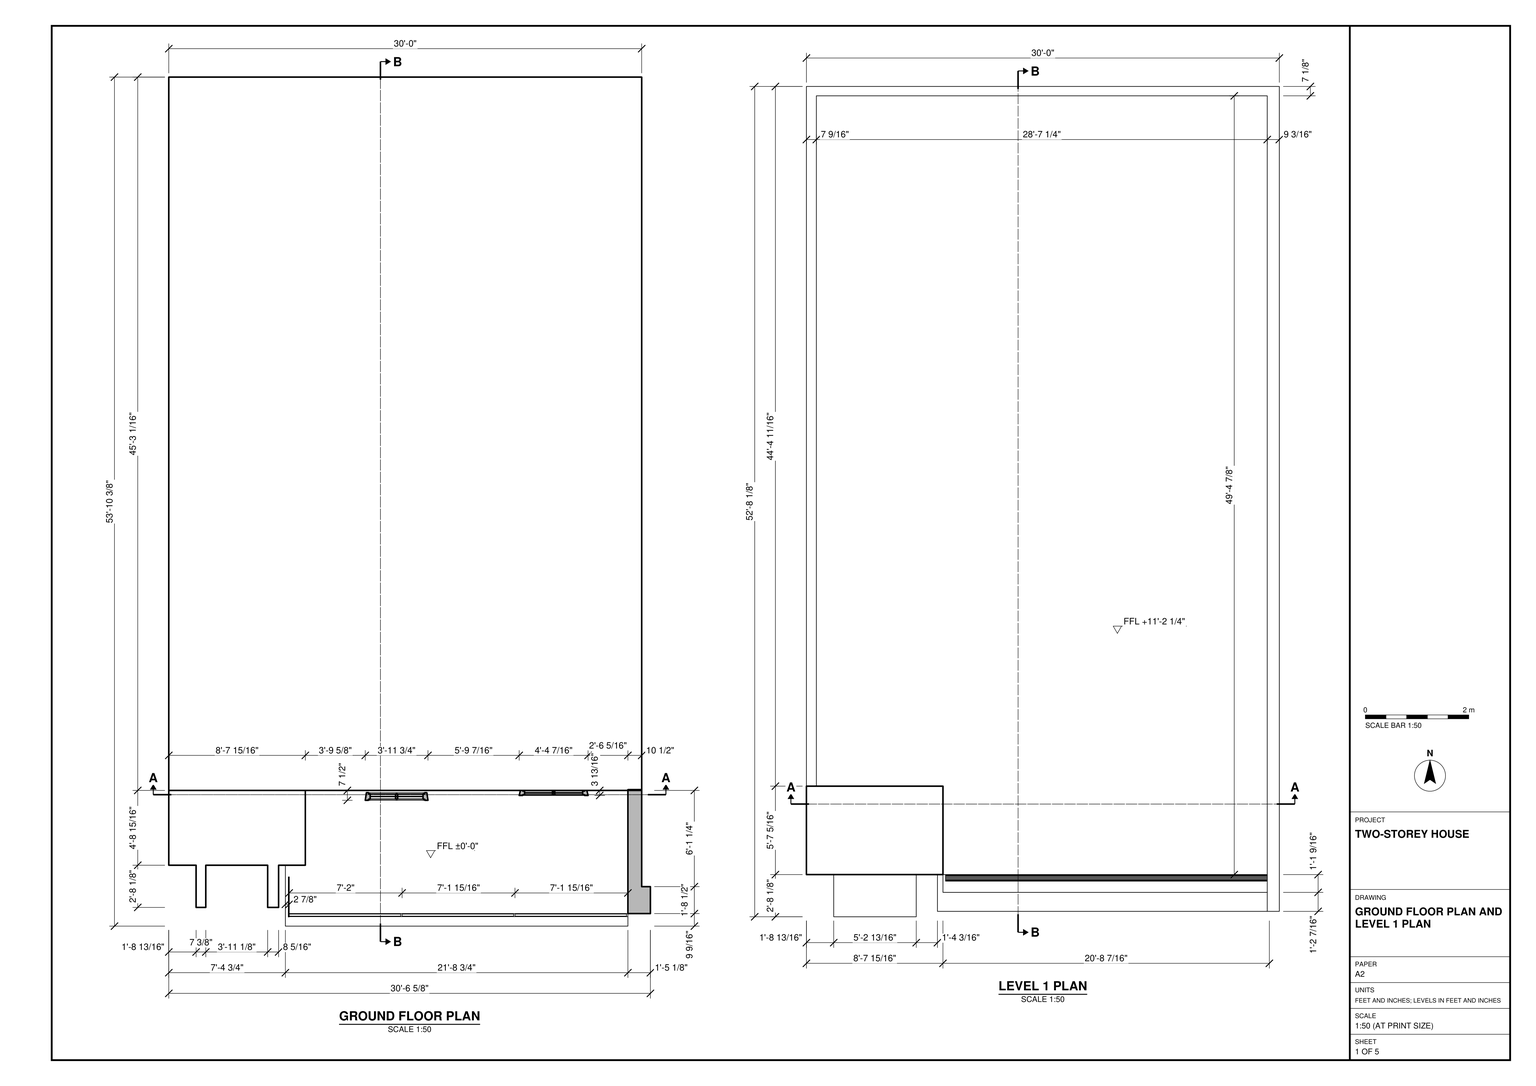
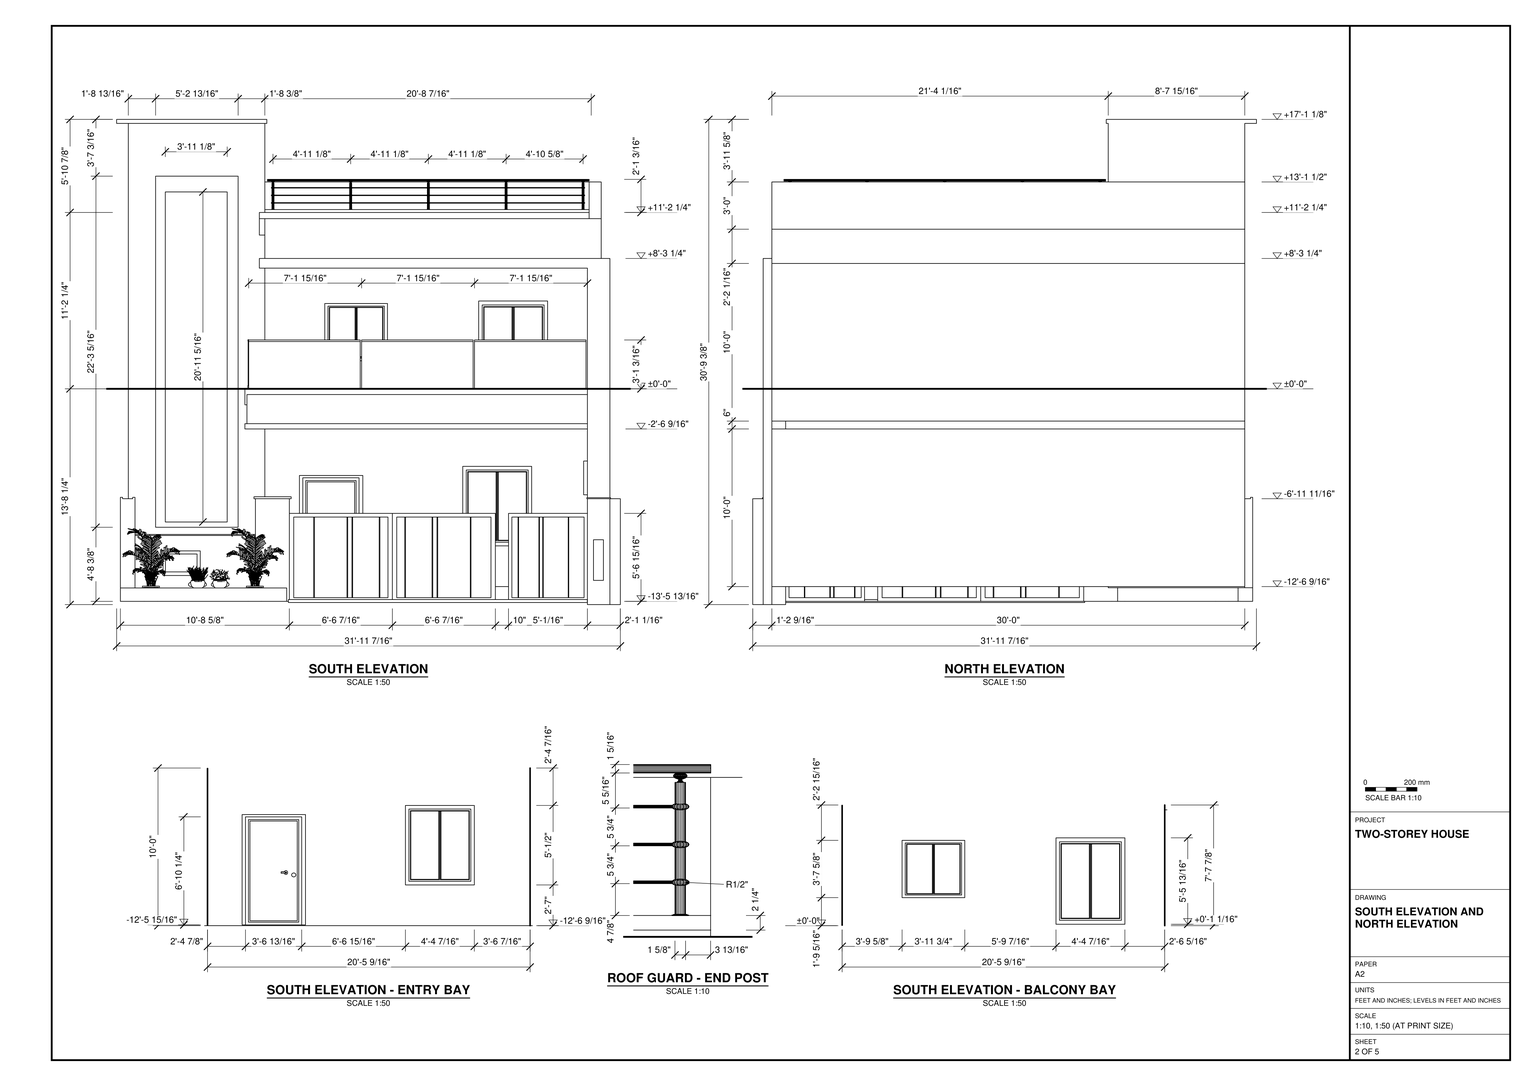
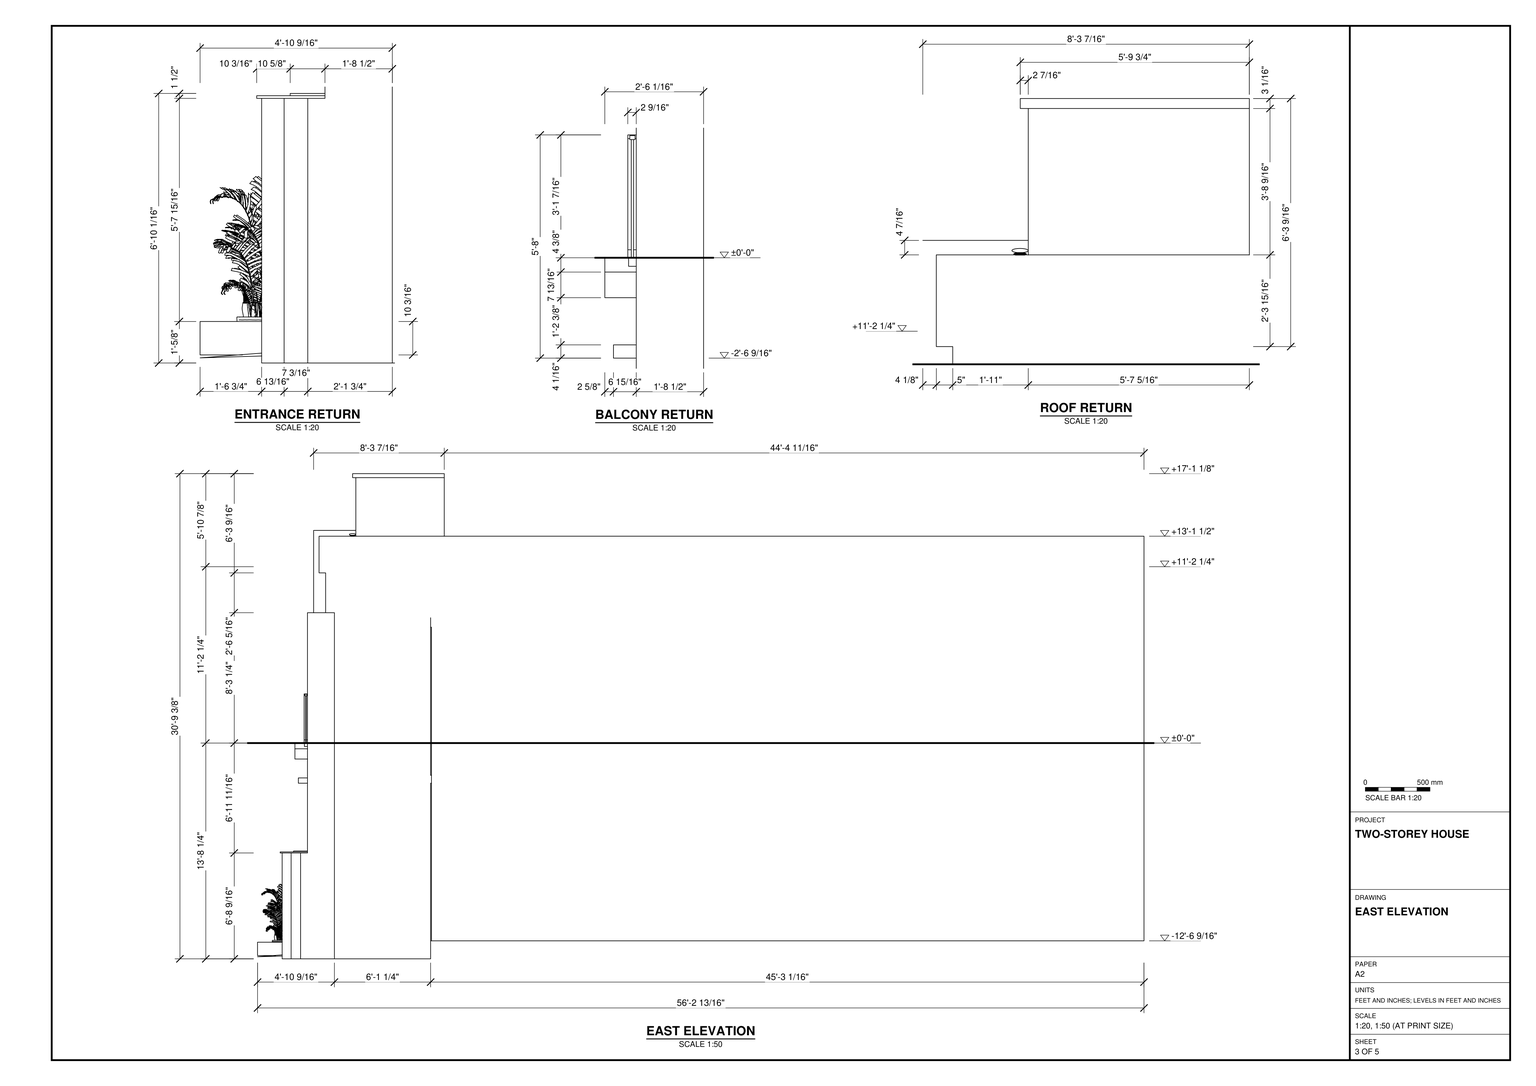
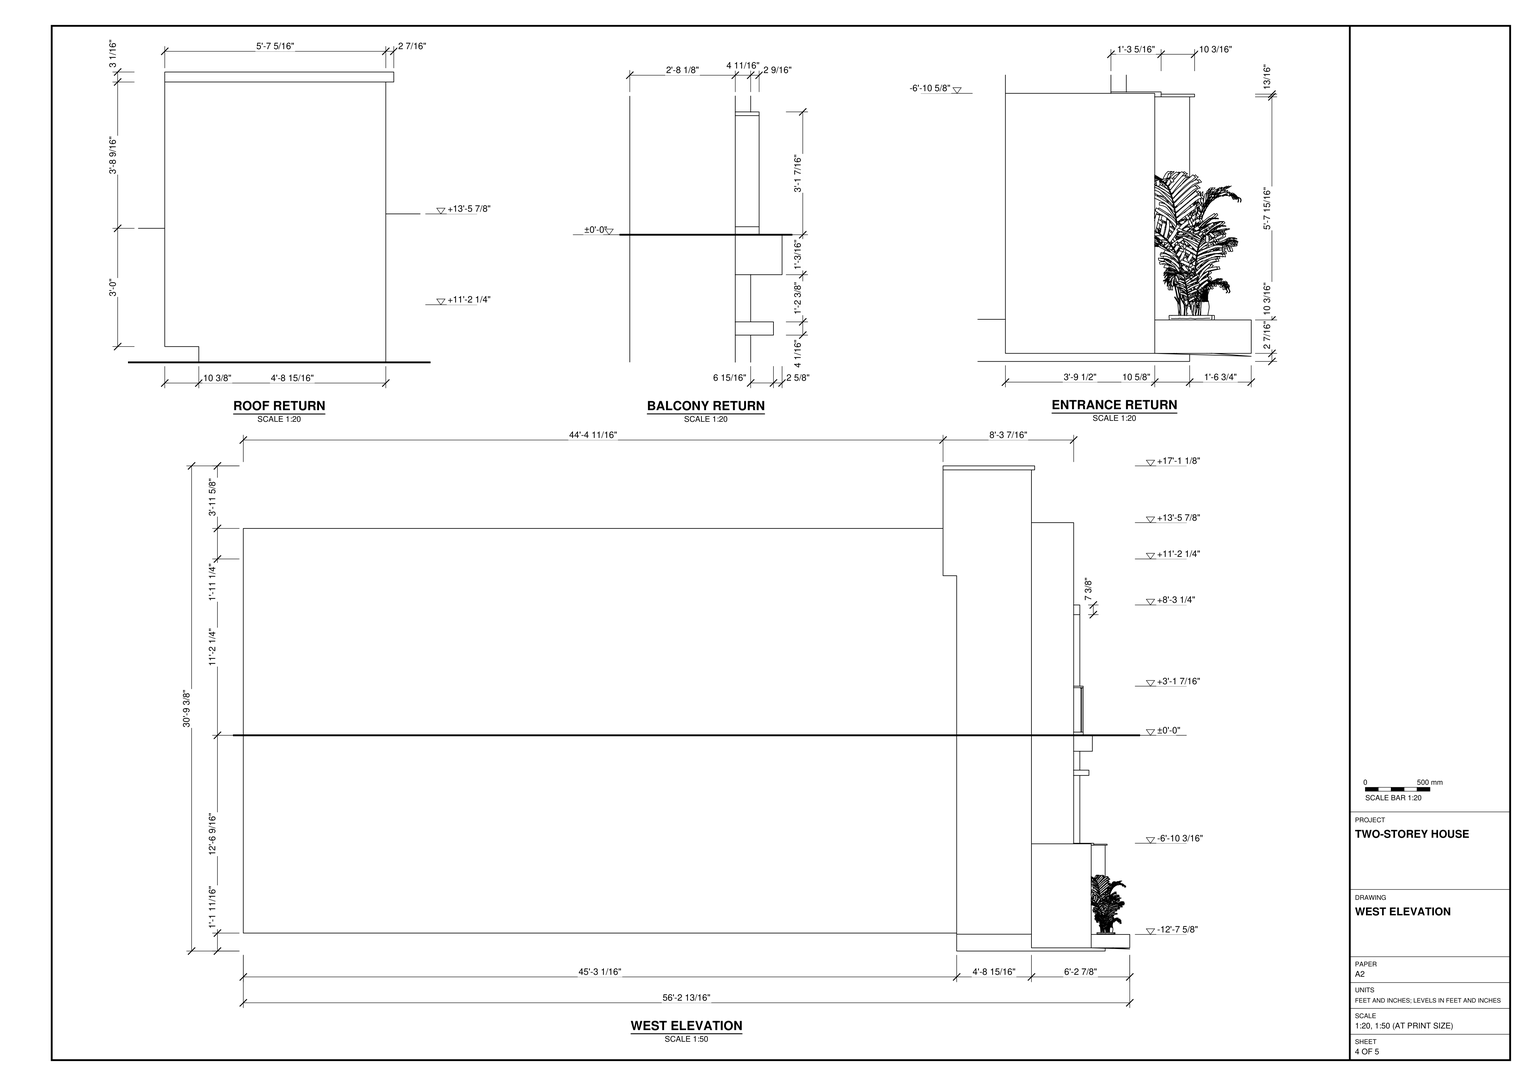
Build the two-storey house in SketchUp from task_files/diagram_01.pdf. Work in feet and inches. Set the overall width to 31'-11 7/16", the front-to-back depth to 56'-2 7/8", and the full height to 30'-9 3/8", including the projections at the entrance and roof. Use the storey levels ±0'-0" and +11'-2 1/4". Follow the elevation datums to place the lower entrance below the balcony.

Use the plans to lay out the long rectangular body, walls at their drawn thicknesses, floor slabs and flat roof with its parapet returns. On the south elevation, model the tall framed bay on the left with its inset panel and projecting cap. Beside it, place the entry door and window behind the panelled gates. Model the balcony slab, glazed guard, framed openings behind the balcony and horizontal roof guard above it. Use the return details to set the depths of these elements. Include the raised planter at the foot of the tall bay.

Keep walls, slabs, roof elements and each furniture or joinery piece shown in separate groups or components, and use components for repeated parts. Decor and loose items such as the entrance plants may be any suitable library components. Save one SketchUp model as output_files/two_storey_house_with_a_glazed_balcony_and_roof_guard.skp.

# SketchUp Ruby script. Lengths in inches.
U = 1.inch
M = Sketchup.active_model
def pt(a) = Geom::Point3d.new(a.map { |v| v * U })
def face(e, loops, mat)
  f = e.add_face(loops[0].map { |a| pt(a) })
  loops[1..].each { |l| e.add_face(l.map { |a| pt(a) }).erase! }
  f.material = f.back_material = mat if mat
  f
end
# faces: each face lists its corners as indices into pts; further lists are holes
def faces(e, pts, list, mat = nil) = list.each { |f| face(e, (f[0].is_a?(Array) ? f : [f]).map { |l| l.map { |i| pts[i] } }, mat) }
# xy, xz, yz: faces in a plane at the given z, y or x. An outline is a flat list of corners, or four numbers for a rectangle; further outlines are holes
def ring(l) = l.size == 4 ? [[l[0], l[1]], [l[2], l[1]], [l[2], l[3]], [l[0], l[3]]] : l.each_slice(2).to_a
def flat(e, list, mat, &to3) = list.each { |f| face(e, (f[0].is_a?(Array) ? f : [f]).map { |l| ring(l).map { |u, v| to3.(u, v) } }, mat) }
def xy(e, z, list, mat = nil) = flat(e, list, mat) { |x, y| [x, y, z] }
def xz(e, y, list, mat = nil) = flat(e, list, mat) { |x, z| [x, y, z] }
def yz(e, x, list, mat = nil) = flat(e, list, mat) { |y, z| [x, y, z] }
def lines(e, pts, list) = list.each { |a, b| e.add_line(pt(pts[a]), pt(pts[b])) }
# prism: a flat outline (further loops are holes) pulled along v
def prism(e, loops, v, mat = nil)
  f = face(e, loops, mat); d = Geom::Vector3d.new(v.map { |x| x * U })
  f.pushpull(f.normal.samedirection?(d) ? d.length : -d.length)
end
def box(e, o, s, mat = nil) = prism(e, [[o, [o[0] + s[0], o[1], o[2]], [o[0] + s[0], o[1] + s[1], o[2]], [o[0], o[1] + s[1], o[2]]]], [0, 0, s[2]], mat)
def at(x, y, z, deg = 0) = Geom::Transformation.translation(pt([x, y, z])) * Geom::Transformation.rotation(ORIGIN, Z_AXIS, deg.degrees)
def axes(o, x, y, z) = Geom::Transformation.new([*x, 0, *y, 0, *z, 0, *pt(o).to_a, 1])
def part(name) = M.definitions.add(name)
# library, detail: a bought-in or finely detailed component or shape, given as its bounding box
def library(name, o, s) = part(name).tap { |d| box(d.entities, o, s) }
def detail(e, o, s) = box(e.add_group.entities, o, s)
def put(e, d, t, mat = nil) = e.add_instance(d, t).tap { |i| i.material = mat if mat }
def group(e, t, mat = nil) = e.add_group.tap { |g| g.transformation = t; g.material = mat if mat }.entities
root = M.entities
M.materials.add("4WA SFSTYD G1").color = [223, 181, 107]
M.materials.add("Aluminum_Anodized_Clear\#1").color = [178, 178, 174]
M.materials.add("Aluminum_Anodized_DarkGray\#1").color = [63, 63, 63]
M.materials.add("[0029_BlanchedAlmond]").color = [255, 235, 205]
M.materials.add("[0135_DarkGray]").color = [81, 81, 81]
M.materials.add("[0136_Charcoal]").color = [35, 35, 35]
M.materials.add("[Aluminum]").color = [179, 179, 179]
M.materials.add("[Color M08]").color = [30, 30, 30]
M.materials.add("[Color M09]").color = [0, 0, 0]
M.materials.add("[Translucent Glass Gray]").color = [128, 128, 128]
M.materials["[Translucent Glass Gray]"].alpha = 0.5
M.materials.add("[Wood Cherry Original]1").color = [152, 86, 42]
M.materials.add("[Wood Floor Parquet]").color = [145, 89, 39]
M.materials.add("[Wood Floor]").color = [155, 105, 61]
M.materials.add("[Wood Lumber ButtJoined]").color = [164, 152, 112]
M.materials.add("[Wood OSB]").color = [240, 195, 122]
M.materials.add("[Wood Veneer 02]").color = [190, 128, 91]
M.materials.add("glass_architectural\#1").color = [217, 197, 188]
M.materials["glass_architectural\#1"].alpha = 0.1
M.materials.add("we3tr gdyr1").color = [92, 92, 92]
c1 = library("trol",[-1.07,-0.37,0],[9.56,15.9,13.04])
c2 = part("Cylinder08")
prism(c2.entities,[[[-163.875,-2.5,0],[-163.95,-2.96,0],[-164.16,-3.38,0],[-164.49,-3.71,0],[-164.91,-3.93,0],[-165.375,-4,0],[-165.84,-3.93,0],[-166.26,-3.71,0],[-166.59,-3.38,0],[-166.8,-2.96,0],[-166.875,-2.5,0],[-166.8,-2.04,0],[-166.59,-1.62,0],[-166.26,-1.29,0],[-165.84,-1.07,0],[-165.375,-1,0],[-164.91,-1.07,0],[-164.49,-1.29,0],[-164.16,-1.62,0],[-163.95,-2.04,0]]],[0,0,78.0625],"4WA SFSTYD G1")
c3 = library("Line04",[-167.3,-4.43,77.97],[3.85,3.86,5.82])
c4 = library("Sphere10",[-167.86,-4.99,61.78],[4.98,4.98,4.14])
c5 = part("Box01")
box(c5.entities,[-176.87,-13.55,-8.45],[462.03,13.55,8.53],"we3tr gdyr1")
c6 = part("Cylinder01")
prism(c6.entities,[[[282.23,-1.73,88.375],[282.23,-2.5,88.5],[282.23,-3.27,88.375],[282.23,-3.97,88.02],[282.23,-4.52,87.47],[282.23,-4.88,86.77],[282.23,-5,86],[282.23,-4.88,85.22],[282.23,-4.52,84.53],[282.23,-3.97,83.97],[282.23,-3.27,83.62],[282.23,-2.5,83.5],[282.23,-1.73,83.62],[282.23,-1.03,83.97],[282.23,-0.48,84.53],[282.23,-0.125,85.22],[282.23,0,86],[282.23,-0.125,86.77],[282.23,-0.48,87.47],[282.23,-1.03,88.02]]],[-455.38,0,0],"4WA SFSTYD G1")
c7 = part("Cylinder03")
prism(c7.entities,[[[-165.34,-2.03,64.49],[-165.34,-1.85,64.3125],[-165.34,-1.74,64.09],[-165.34,-1.7,63.84],[-165.34,-1.74,63.59],[-165.34,-1.85,63.37],[-165.34,-2.03,63.19],[-165.34,-2.25,63.08],[-165.34,-2.5,63.04],[-165.34,-2.75,63.08],[-165.34,-2.97,63.19],[-165.34,-3.15,63.37],[-165.34,-3.26,63.59],[-165.34,-3.3,63.84],[-165.34,-3.26,64.09],[-165.34,-3.15,64.3125],[-165.34,-2.97,64.49],[-165.34,-2.75,64.6],[-165.34,-2.5,64.64],[-165.34,-2.25,64.6]]],[438.09,0,0],"4WA SFSTYD G1")
c8 = library("Line08",[-167.875,-5,0],[5,5,0.9])
c9 = part("skp246")
put(c9.entities,c2,at(0,0,0))
put(c9.entities,c3,at(0,0,0))
put(c9.entities,c4,at(0,0,0))
put(c9.entities,c5,at(0,0,0))
put(c9.entities,c6,at(0,0,0))
put(c9.entities,c7,at(0,0,0))
put(c9.entities,c8,at(0,0,0))
put(c9.entities,c4,at(0,0,-22.16))
put(c9.entities,c4,at(0,0,-44.3))
put(c9.entities,c7,at(0,0,-22.14))
put(c9.entities,c7,at(0,0,-44.28))
put(c9.entities,c4,at(110,0,-44.3))
put(c9.entities,c4,at(110,0,-22.16))
put(c9.entities,c4,at(110,0,0))
put(c9.entities,c2,at(110,0,0))
put(c9.entities,c8,at(110,0,0))
put(c9.entities,c3,at(110,0,0))
put(c9.entities,c4,at(220,0,-22.16))
put(c9.entities,c3,at(220,0,0))
put(c9.entities,c4,at(220,0,0))
put(c9.entities,c4,at(220,0,-44.3))
put(c9.entities,c2,at(220,0,0))
put(c9.entities,c8,at(220,0,0))
put(c9.entities,c3,at(330,0,0))
put(c9.entities,c4,at(330,0,-44.3))
put(c9.entities,c4,at(330,0,-22.16))
put(c9.entities,c8,at(330,0,0))
put(c9.entities,c2,at(330,0,0))
put(c9.entities,c4,at(330,0,0))
put(c9.entities,c4,at(438.97,0,-22.16))
put(c9.entities,c4,at(438.97,0,0))
put(c9.entities,c4,at(438.97,0,-44.3))
put(c9.entities,c8,at(438.97,0,0))
put(c9.entities,c2,at(438.97,0,0))
put(c9.entities,c3,at(438.97,0,0))
c10 = part("Railing1 (1)")
put(c10.entities,c9,at(176.87,13.55,8.45))
c11 = part("window")
xy(c11.entities,-137.04,[[3.3,-12.46,3.83,49.56]],"[Wood Veneer 02]")
xy(c11.entities,-136.95,[[0,-12.36,0.53,49.45]],"[Wood Veneer 02]")
xy(c11.entities,-135.68,[[3.08,-10.98,3.3,18.15],[3.08,18.94,3.3,48.07]],"[Color M09]")
xy(c11.entities,-135.5,[[0.53,-10.78,0.74,18.05],[0.53,19.04,0.74,47.88]],"[Color M09]")
xy(c11.entities,-135.27,[[0.74,-10.54,1.91,17.37],[1.91,-10.54,3.08,17.37],[0.74,19.73,1.91,47.63],[1.91,19.73,3.08,47.63]],"[Color M09]")
xy(c11.entities,-74.87,[[1.91,17.37,3.08,19.73],[0.74,19.73,1.91,47.63]])
xy(c11.entities,-74.87,[[0.74,-10.54,1.91,17.37],[1.91,-10.54,3.08,17.37],[1.91,19.73,3.08,47.63]],"[Color M09]")
xy(c11.entities,-74.65,[[0.53,19.04,0.74,47.88]])
xy(c11.entities,-74.65,[[0.53,-10.78,0.74,18.05]],"[Color M09]")
xy(c11.entities,-74.47,[[3.08,18.15,3.3,18.94]])
xy(c11.entities,-74.47,[[3.08,-10.98,3.3,18.15],[3.08,18.94,3.3,48.07]],"[Color M09]")
xy(c11.entities,-73.2,[[0,-12.36,0.53,49.45]],"[Wood Veneer 02]")
xy(c11.entities,-73.1,[[3.3,-12.46,3.83,49.56]],"[Wood Veneer 02]")
xy(c11.entities,3.5,[[3.3,3.5,3.83,65.52]],"[Wood Veneer 02]")
xy(c11.entities,3.6,[[0,3.6,0.53,65.41]],"[Wood Veneer 02]")
xy(c11.entities,4.98,[[3.08,4.98,3.3,34.12],[3.08,34.9,3.3,64.04]],"[Color M09]")
xy(c11.entities,5.18,[[0.53,5.18,0.74,34.01],[0.53,35,0.74,63.84]],"[Color M09]")
xy(c11.entities,5.42,[[0.74,5.42,1.91,33.33],[1.91,5.42,3.08,33.33],[0.74,35.69,1.91,63.59],[1.91,35.69,3.08,63.59]],"[Color M09]")
xy(c11.entities,25.89,[[6.71,-150.99,7.52,-94.56]],"[Wood Veneer 02]")
xy(c11.entities,25.96,[[1.71,-150.9,2.52,-94.65]],"[Wood Veneer 02]")
xy(c11.entities,26.87,[[6.39,-149.64,6.71,-123.13],[6.39,-122.42,6.71,-95.9]],"[Color M09]")
xy(c11.entities,27,[[2.52,-149.46,2.84,-123.22],[2.52,-122.32,2.84,-96.08]],"[Color M09]")
xy(c11.entities,27.16,[[2.84,-149.24,4.61,-123.85],[4.61,-149.24,6.39,-123.85],[2.84,-121.7,4.61,-96.31],[4.61,-121.7,6.39,-96.31]],"[Color M09]")
xy(c11.entities,70.69,[[4.61,-123.85,6.39,-121.7],[2.84,-121.7,4.61,-96.31]])
xy(c11.entities,70.69,[[2.84,-149.24,4.61,-123.85],[4.61,-149.24,6.39,-123.85],[4.61,-121.7,6.39,-96.31]],"[Color M09]")
xy(c11.entities,70.85,[[2.52,-122.32,2.84,-96.08]])
xy(c11.entities,70.85,[[2.52,-149.46,2.84,-123.22]],"[Color M09]")
xy(c11.entities,70.98,[[6.39,-123.13,6.71,-122.42]])
xy(c11.entities,70.98,[[6.39,-149.64,6.71,-123.13],[6.39,-122.42,6.71,-95.9]],"[Color M09]")
xy(c11.entities,71.07,[[1.91,33.33,3.08,35.69],[0.74,35.69,1.91,63.59]])
xy(c11.entities,71.07,[[0.74,5.42,1.91,33.33],[1.91,5.42,3.08,33.33],[1.91,35.69,3.08,63.59]],"[Color M09]")
xy(c11.entities,71.32,[[0.53,35,0.74,63.84]])
xy(c11.entities,71.32,[[0.53,5.18,0.74,34.01]],"[Color M09]")
xy(c11.entities,71.52,[[3.08,34.12,3.3,34.9]])
xy(c11.entities,71.52,[[3.08,4.98,3.3,34.12],[3.08,34.9,3.3,64.04]],"[Color M09]")
xy(c11.entities,71.9,[[1.71,-150.9,2.52,-94.65]],"[Wood Veneer 02]")
xy(c11.entities,71.97,[[6.71,-150.99,7.52,-94.56]],"[Wood Veneer 02]")
xy(c11.entities,72.9,[[0,3.6,0.53,65.41]],"[Wood Veneer 02]")
xy(c11.entities,73,[[3.3,3.5,3.83,65.52]],"[Wood Veneer 02]")
xz(c11.entities,-150.99,[[6.71,25.89,7.52,71.97]],"[Wood Veneer 02]")
xz(c11.entities,-150.9,[[1.71,25.96,2.52,71.9]],"[Wood Veneer 02]")
xz(c11.entities,-149.64,[[6.39,26.87,6.71,70.98]],"[Color M09]")
xz(c11.entities,-149.46,[[2.52,27,2.84,70.85]],"[Color M09]")
xz(c11.entities,-149.24,[[2.84,27.16,4.61,70.69],[4.61,27.16,6.39,70.69]],"[Color M09]")
xz(c11.entities,-123.85,[[2.84,27.16,6.39,70.69]],"[Color M09]")
xz(c11.entities,-123.22,[[2.52,27,2.84,70.85]],"[Wood Floor]")
xz(c11.entities,-123.13,[[6.39,26.87,6.71,70.98]],"[Color M09]")
xz(c11.entities,-122.42,[[6.39,26.87,6.71,56.14],[6.39,56.14,6.71,70.98]],"[Color M09]")
xz(c11.entities,-122.32,[[2.52,27,2.84,70.85]],"[Color M09]")
xz(c11.entities,-121.7,[[2.84,27.16,6.39,70.69]],"[Color M09]")
xz(c11.entities,-96.31,[[2.84,27.16,4.61,70.69],[4.61,27.16,6.39,70.69]],"[Wood Floor]")
xz(c11.entities,-96.08,[[2.52,27,2.84,70.85]],"[Wood Floor]")
xz(c11.entities,-95.9,[[6.39,26.87,6.71,70.98]],"[Color M09]")
xz(c11.entities,-94.65,[[1.71,25.96,2.52,71.9]],"[Wood Veneer 02]")
xz(c11.entities,-94.56,[[6.71,25.89,7.52,71.97]],"[Wood Veneer 02]")
xz(c11.entities,-12.46,[[3.3,-137.04,3.83,-73.1]],"[Wood Veneer 02]")
xz(c11.entities,-12.36,[[0,-136.95,0.53,-73.2]],"[Wood Veneer 02]")
xz(c11.entities,-10.98,[[3.08,-135.68,3.3,-74.47]],"[Color M09]")
xz(c11.entities,-10.78,[[0.53,-135.5,0.74,-74.65]],"[Color M09]")
xz(c11.entities,-10.54,[[0.74,-135.27,1.91,-74.87],[1.91,-135.27,3.08,-74.87]],"[Color M09]")
xz(c11.entities,3.5,[[3.3,3.5,3.83,73]],"[Wood Veneer 02]")
xz(c11.entities,3.6,[[0,3.6,0.53,72.9]],"[Wood Veneer 02]")
xz(c11.entities,4.98,[[3.08,4.98,3.3,71.52]],"[Color M09]")
xz(c11.entities,5.18,[[0.53,5.18,0.74,71.32]],"[Color M09]")
xz(c11.entities,5.42,[[0.74,5.42,1.91,71.07],[1.91,5.42,3.08,71.07]],"[Color M09]")
xz(c11.entities,17.37,[[0.74,-135.27,3.08,-74.87]],"[Color M09]")
xz(c11.entities,18.05,[[0.53,-135.5,0.74,-74.65]],"[Wood Floor]")
xz(c11.entities,18.15,[[3.08,-135.68,3.3,-74.47]],"[Color M09]")
xz(c11.entities,18.94,[[3.08,-135.68,3.3,-95.07],[3.08,-95.07,3.3,-74.47]],"[Color M09]")
xz(c11.entities,19.04,[[0.53,-135.5,0.74,-74.65]],"[Color M09]")
xz(c11.entities,19.73,[[0.74,-135.27,3.08,-74.87]],"[Color M09]")
xz(c11.entities,33.33,[[0.74,5.42,3.08,71.07]],"[Color M09]")
xz(c11.entities,34.01,[[0.53,5.18,0.74,71.32]],"[Wood Floor]")
xz(c11.entities,34.12,[[3.08,4.98,3.3,71.52]],"[Color M09]")
xz(c11.entities,34.9,[[3.08,4.98,3.3,49.125],[3.08,49.125,3.3,71.52]],"[Color M09]")
xz(c11.entities,35,[[0.53,5.18,0.74,71.32]],"[Color M09]")
xz(c11.entities,35.69,[[0.74,5.42,3.08,71.07]],"[Color M09]")
xz(c11.entities,47.63,[[0.74,-135.27,1.91,-74.87],[1.91,-135.27,3.08,-74.87]],"[Wood Floor]")
xz(c11.entities,47.88,[[0.53,-135.5,0.74,-74.65]],"[Wood Floor]")
xz(c11.entities,48.07,[[3.08,-135.68,3.3,-74.47]],"[Color M09]")
xz(c11.entities,49.45,[[0,-136.95,0.53,-73.2]],"[Wood Veneer 02]")
xz(c11.entities,49.56,[[3.3,-137.04,3.83,-73.1]],"[Wood Veneer 02]")
xz(c11.entities,63.59,[[0.74,5.42,1.91,71.07],[1.91,5.42,3.08,71.07]],"[Wood Floor]")
xz(c11.entities,63.84,[[0.53,5.18,0.74,71.32]],"[Wood Floor]")
xz(c11.entities,64.04,[[3.08,4.98,3.3,71.52]],"[Color M09]")
xz(c11.entities,65.41,[[0,3.6,0.53,72.9]],"[Wood Veneer 02]")
xz(c11.entities,65.52,[[3.3,3.5,3.83,73]],"[Wood Veneer 02]")
yz(c11.entities,0,[[[-14.72,-139.12,51.82,-71.02],[-12.36,-136.95,49.45,-73.2]],[[1.24,1.24,67.78,75.26],[3.6,3.6,65.41,72.9]]],"[Wood Veneer 02]")
yz(c11.entities,0.53,[[[-12.36,-136.95,49.45,-73.2],[19.04,-135.5,47.88,-74.65],[-10.78,-135.5,18.05,-74.65]],[[3.6,3.6,65.41,72.9],[5.18,5.18,34.01,71.32],[35,5.18,63.84,71.32]]],"[Color M09]")
yz(c11.entities,0.74,[[18.05,-135.5,19.04,-135.27],[18.05,-135.27,19.04,-74.87],[18.05,-74.87,19.04,-74.65],[34.01,5.18,35,5.42],[34.01,5.42,35,71.07],
  [34.01,71.07,35,71.32]])
yz(c11.entities,0.74,[[[-10.78,-135.5,18.05,-74.65],[-10.54,-135.27,17.37,-74.87]],[[19.04,-135.5,47.88,-74.65],[19.73,-135.27,47.63,-74.87]],[[5.18,5.18,34.01,71.32],[5.42,5.42,33.33,71.07]],[[35,5.18,63.84,71.32],[35.69,5.42,63.59,71.07]]],"[Color M09]")
yz(c11.entities,1.71,[[[-153.05,24.39,-92.5,73.46],[-150.9,25.96,-94.65,71.9]]],"[Wood Veneer 02]")
yz(c11.entities,1.91,[[-10.54,-135.27,47.63,-74.87],[5.42,5.42,63.59,71.07]],"[Translucent Glass Gray]")
yz(c11.entities,2.52,[[[-150.9,25.96,-94.65,71.9],[-122.32,27,-96.08,70.85],[-149.46,27,-123.22,70.85]]],"[Color M09]")
yz(c11.entities,2.84,[[-123.22,27,-122.32,27.16],[-123.22,27.16,-122.32,70.69],[-123.22,70.69,-122.32,70.85]])
yz(c11.entities,2.84,[[[-149.46,27,-123.22,70.85],[-149.24,27.16,-123.85,70.69]],[[-122.32,27,-96.08,70.85],[-121.7,27.16,-96.31,70.69]]],"[Color M09]")
yz(c11.entities,3.08,[[18.15,-74.87,18.94,-74.47],[34.12,71.07,34.9,71.52]])
yz(c11.entities,3.08,[[[-10.98,-135.68,18.15,-74.47],[-10.54,-135.27,17.37,-74.87]],[[18.94,-135.68,48.07,-74.47],[19.73,-135.27,47.63,-74.87]],[[4.98,4.98,34.12,71.52],[5.42,5.42,33.33,71.07]],[[34.9,4.98,64.04,71.52],[35.69,5.42,63.59,71.07]]],"[Color M09]")
yz(c11.entities,3.3,[[[-12.46,-137.04,49.56,-73.1],[-10.98,-135.68,18.15,-74.47],[18.94,-135.68,48.07,-74.47]],[[3.5,3.5,65.52,73],[34.9,4.98,64.04,71.52],[4.98,4.98,34.12,71.52]]],"[Color M09]")
yz(c11.entities,3.83,[[[-15.96,-140.26,53.06,-69.88],[-12.46,-137.04,49.56,-73.1]],[[0,0,69.02,76.5],[3.5,3.5,65.52,73]]],"[Wood Veneer 02]")
yz(c11.entities,4.61,[[-149.24,27.16,-96.31,70.69]],"[Translucent Glass Gray]")
yz(c11.entities,6.39,[[-123.13,70.69,-122.42,70.98]])
yz(c11.entities,6.39,[[[-149.64,26.87,-123.13,70.98],[-149.24,27.16,-123.85,70.69]],[[-122.42,26.87,-95.9,70.98],[-121.7,27.16,-96.31,70.69]]],"[Color M09]")
yz(c11.entities,6.71,[[[-150.99,25.89,-94.56,71.97],[-149.64,26.87,-123.13,70.98],[-122.42,26.87,-95.9,70.98]]],"[Color M09]")
yz(c11.entities,7.52,[[[-154.18,23.57,-91.37,74.29],[-150.99,25.89,-94.56,71.97]]],"[Wood Veneer 02]")
# 3 loose lines left out
p = [[0,-14.72,-139.12],[3.83,-15.96,-140.26],[3.83,-15.96,-69.88],[0,-14.72,-71.02],[0,51.82,-139.12],[3.83,53.06,-140.26],
  [0,51.82,-71.02],[3.83,53.06,-69.88],[0,1.24,1.24],[3.83,0,0],[3.83,0,76.5],[0,1.24,75.26],
  [0,67.78,1.24],[3.83,69.02,0],[0,67.78,75.26],[3.83,69.02,76.5],[1.71,-153.05,24.39],[1.71,-92.5,24.39],
  [7.52,-91.37,23.57],[7.52,-154.18,23.57],[7.52,-154.18,74.29],[1.71,-153.05,73.46],[1.71,-92.5,73.46],[7.52,-91.37,74.29]]
faces(c11.entities,p,[[0,1,2,3],[8,9,10,11],[16,19,20,21]],"[Wood Floor]")
faces(c11.entities,p,[[0,4,5,1],[8,12,13,9],[16,17,18,19]])
faces(c11.entities,p,[[5,4,6,7],[6,3,2,7],[13,12,14,15],[18,17,22,23],[22,21,20,23],[14,11,10,15]],"[Wood Veneer 02]")
c12 = part("GLASS")
box(c12.entities,[0,0,0],[48,0.8,36])
c13 = part("STEEL BAR")
box(c13.entities,[0,-0.1,0],[48,1.8,1.2])
c14 = part("LOWER PART")
box(c14.entities,[0,-0.6,0],[48.6,2.6,2.6])
c15 = part("BALCONY GLASS ")
put(c15.entities,c12,at(0,0.9,2.6),"glass_architectural\#1")
put(c15.entities,c13,at(0,0.5,38.6),"Aluminum_Anodized_DarkGray\#1")
put(c15.entities,c14,at(0,0.6,0),"Aluminum_Anodized_Clear\#1")
c16 = part("NO 3")
put(c16.entities,c15,at(0,0,0))
put(c16.entities,c15,at(48.6,0,0))
put(c16.entities,c15,at(97.2,0,0))
c17 = part("Door lever handle")
xy(c17.entities,0.89,[[5.42,1.98,1.2,2,1.2,2.25,5.42,2.23]],"[Aluminum]")
xy(c17.entities,1.84,[[5.42,1.98,5.42,2.23,1.25,2.25,1.25,2]],"[Aluminum]")
xy(c17.entities,1.85,[[1.28,0.75,1.41,2.25]],"[Wood Cherry Original]1")
xz(c17.entities,0.75,[[[1.4375,0,1.81,0.05,2.16,0.19,2.45,0.42,2.68,0.72,2.83,1.07,2.875,1.4375,2.83,1.81,2.68,2.16,2.45,2.45,2.16,2.68,1.81,2.83,1.4375,2.875,1.07,2.83,0.72,2.68,0.42,2.45,0.19,2.16,0.05,1.81,0,1.4375,0.05,1.07,0.19,0.72,0.42,0.42,0.72,0.19,1.07,0.05],[1.33,0.87,1.2,0.89,1.09,0.95,0.99,1.04,0.92,1.15,0.88,1.27,0.875,1.4,0.9,1.52,0.96,1.64,1.05,1.74,1.16,1.81,1.28,1.85,1.41,1.85,1.53,1.83,1.65,1.77,1.74,1.68,1.8125,1.57,1.85,1.45,1.86,1.32,1.83,1.2,1.78,1.08,1.69,0.99,1.58,0.91,1.46,0.875]]],"[Wood Cherry Original]1")
xz(c17.entities,2.25,[[1.33,0.87,1.46,0.875,1.58,0.91,1.69,0.99,1.78,1.08,1.83,1.2,1.86,1.32,1.85,1.45,1.8125,1.57,1.74,1.68,1.65,1.77,1.53,1.83,1.41,1.85,1.28,1.85,1.25,1.84,1.2,1.82,1.2,0.89],[1.2,0.89,1.2,1.82,1.16,1.81,1.05,1.74,0.96,1.64,0.9,1.52,0.875,1.4,0.88,1.27,0.92,1.15,0.99,1.04,1.09,0.95]],"[Wood Cherry Original]1")
yz(c17.entities,5.42,[[1.98,0.89,2.23,1.84]],"[Aluminum]")
p = [[0.72,0,0.19],[1.07,0,0.05],[1.07,0.75,0.05],[0.72,0.75,0.19],[1.4375,0,0],[1.4375,0.75,0],
  [1.81,0,0.05],[1.81,0.75,0.05],[2.16,0,0.19],[2.16,0.75,0.19],[0.42,0,0.42],[0.42,0.75,0.42],
  [2.45,0,0.42],[2.45,0.75,0.42],[0.19,0,0.72],[0.19,0.75,0.72],[2.68,0,0.72],[2.68,0.75,0.72],
  [0.05,0,1.07],[0.05,0.75,1.07],[2.83,0,1.07],[2.83,0.75,1.07],[1.09,0.75,0.95],[1.2,0.75,0.89],
  [1.2,2,0.89],[1.2,2.25,0.89],[1.09,2.25,0.95],[1.33,0.75,0.87],[1.33,2.25,0.87],[1.46,0.75,0.875],
  [1.46,2.25,0.875],[1.58,0.75,0.91],[1.58,2.25,0.91],[1.69,0.75,0.99],[1.69,2.25,0.99],[1.25,2.25,1.84],
  [5.42,2.23,1.84],[5.42,2.23,0.89],[1.2,2.25,1.82],[0.92,0.75,1.15],[0.99,0.75,1.04],[0.99,2.25,1.04],
  [0.92,2.25,1.15],[1.78,0.75,1.08],[1.78,2.25,1.08],[0,0,1.4375],[0,0.75,1.4375],[2.875,0,1.4375],
  [2.875,0.75,1.4375],[0.88,0.75,1.27],[0.88,2.25,1.27],[1.83,0.75,1.2],[1.83,2.25,1.2],[1.86,0.75,1.32],
  [1.86,2.25,1.32],[0.875,0.75,1.4],[0.875,2.25,1.4],[1.85,0.75,1.45],[1.85,2.25,1.45],[0.05,0,1.81],
  [0.05,0.75,1.81],[2.83,0,1.81],[2.83,0.75,1.81],[0.9,0.75,1.52],[0.9,2.25,1.52],[0.96,0.75,1.64],
  [0.96,2.25,1.64],[1.8125,0.75,1.57],[1.8125,2.25,1.57],[1.05,0.75,1.74],[1.05,2.25,1.74],[1.74,0.75,1.68],
  [1.74,2.25,1.68],[1.16,0.75,1.81],[1.16,2.25,1.81],[1.65,0.75,1.77],[1.65,2.25,1.77],[0.19,0,2.16],
  [0.19,0.75,2.16],[2.68,0,2.16],[2.68,0.75,2.16],[1.28,0.75,1.85],[1.28,2.25,1.85],[1.53,0.75,1.83],
  [1.41,0.75,1.85],[1.41,2.25,1.85],[1.53,2.25,1.83],[0.42,0,2.45],[0.42,0.75,2.45],[2.45,0,2.45],
  [2.45,0.75,2.45],[0.72,0,2.68],[0.72,0.75,2.68],[2.16,0,2.68],[2.16,0.75,2.68],[1.07,0,2.83],
  [1.07,0.75,2.83],[1.81,0,2.83],[1.81,0.75,2.83],[1.4375,0,2.875],[1.4375,0.75,2.875]]
faces(c17.entities,p,[[0,1,2,3],[1,4,5,2],[4,6,7,5],[6,8,9,7],[10,0,3,11],[8,12,13,9],[14,10,11,15],[12,16,17,13],
  [18,14,15,19],[16,20,21,17],[22,23,24,25,26],[23,27,28,25,24],[27,29,30,28],[29,31,32,30],[31,33,34,32],[39,40,41,42],
  [40,22,26,41],[33,43,44,34],[45,18,19,46],[20,47,48,21],[49,39,42,50],[43,51,52,44],[51,53,54,52],[55,49,50,56],
  [53,57,58,54],[59,45,46,60],[47,61,62,48],[63,55,56,64],[65,63,64,66],[57,67,68,58],[69,65,66,70],[67,71,72,68],
  [73,69,70,74],[71,75,76,72],[77,59,60,78],[61,79,80,62],[81,73,74,38,35,82],[83,84,85,86],[75,83,86,76],[87,77,78,88],
  [79,89,90,80],[91,87,88,92],[89,93,94,90],[95,91,92,96],[93,97,98,94],[99,95,96,100],[97,99,100,98]],"[Wood Cherry Original]1")
faces(c17.entities,p,[[35,36,37,25,38]],"[Aluminum]")
c18 = part("Hinged door")
xy(c18.entities,1.35,[[-7.78,3.1,39.03,10.1]],"[Aluminum]")
xy(c18.entities,3.37,[[-5.3125,3.1,36.5625,7.23],[-5.3125,7.23,36.5625,10.1]],"[Wood Cherry Original]1")
xy(c18.entities,4.38,[[-4.08,6.85,35.33,7.23]],"[Wood Cherry Original]1")
xy(c18.entities,77.04,[[-4.08,6.85,35.33,7.23]],"[Wood Cherry Original]1")
xy(c18.entities,78.05,[[-5.3125,3.1,36.5625,7.23],[-5.3125,7.23,36.5625,10.1]],"[Wood Cherry Original]1")
xy(c18.entities,80.07,[[-7.78,3.1,39.03,10.1]],"[Wood Cherry Original]1")
xz(c18.entities,3.1,[[[-7.78,1.35,39.03,80.07],[-5.3125,3.37,36.5625,78.05]]],"[Wood Cherry Original]1")
xz(c18.entities,6.85,[[[-4.08,4.38,35.33,77.04],[-1.15,42.21,-1.61,42.26,-2.04,42.4,-2.4,42.63,-2.68,42.93,-2.86,43.28,-2.92,43.66,-2.86,44.03,-2.68,44.38,-2.4,44.68,-2.04,44.91,-1.61,45.06,-1.15,45.11,-0.69,45.06,-0.27,44.91,0.1,44.68,0.38,44.38,0.56,44.03,0.62,43.66,0.56,43.28,0.38,42.93,0.1,42.63,-0.27,42.4,-0.69,42.26]]],"[Wood Cherry Original]1")
xz(c18.entities,7.23,[[[-5.3125,3.37,36.5625,78.05],[-4.08,4.38,35.33,77.04]]],"[Wood Cherry Original]1")
xz(c18.entities,10.1,[[[-7.78,1.35,39.03,80.07],[-5.3125,3.37,36.5625,78.05]]],"[Wood Cherry Original]1")
yz(c18.entities,-7.78,[[3.1,1.35,10.1,80.07]],"[Wood Cherry Original]1")
yz(c18.entities,-5.3125,[[3.1,3.37,7.23,78.05],[7.23,3.37,10.1,78.05]],"[Wood Cherry Original]1")
yz(c18.entities,-4.08,[[6.85,4.38,7.23,77.04]],"[Wood Cherry Original]1")
yz(c18.entities,5.15,[[5.75,41.38,6,42.3]])
yz(c18.entities,35.33,[[6.85,4.38,7.23,77.04]],"[Wood Cherry Original]1")
yz(c18.entities,36.5625,[[3.1,3.37,7.23,78.05],[7.23,3.37,10.1,78.05]],"[Wood Cherry Original]1")
yz(c18.entities,39.03,[[3.1,1.35,10.1,80.07]],"[Wood Cherry Original]1")
# 2 loose lines left out
p = [[9.36,5.73,42.32],[5.19,5.75,42.32],[5.15,5.75,42.3],[5.15,5.75,41.38],[5.15,5.75,41.38],[9.36,5.73,41.38],
  [5.19,6,42.32],[5.15,6,42.3]]
faces(c18.entities,p,[[0,1,2,3,4,5],[6,7,2,1]])
put(c18.entities,c17,at(3.94,3.75,40.48))
put(c18.entities,c17,axes([3.94,3.75,43.36],[1,0,0],[0,-1,0],[0,0,-1]))
c19 = part("Group\#102")
g1 = group(c19.entities,at(0,0,0))
prism(g1,[[[0,3,72],[70.5,3,72],[70.5,3,0],[0,3,0]],[[67.5,3,3],[67.5,3,69],[3,3,69],[3,3,3]]],[0,-3,0])
c20 = part("Group\#135")
box(c20.entities,[0,0,0],[0.5,1,66])
c21 = part("Group\#148")
box(c21.entities,[0,-1,0],[5.5,1,66])
box(c21.entities,[50.84,-1,0],[13.66,1,66])
box(c21.entities,[28.06,-1,0],[22.28,1,66])
box(c21.entities,[24.66,-1,0],[2.9,1,66])
box(c21.entities,[6,-1,0],[18.16,1,66])
c22 = part("Framed window panels")
g2 = group(c22.entities,at(70.5,0,0),"[Color M08]")
put(g2,c19,axes([70.5,0,0],[-1,0,0],[0,1,0],[0,0,1]))
g3 = group(g2,at(3,2,3))
g4 = group(g3,at(0,-1,0))
box(g4,[0,0,0],[5.5,1,66])
box(g4,[50.84,0,0],[13.66,1,66])
box(g4,[28.06,0,0],[22.28,1,66])
box(g4,[24.66,0,0],[2.9,1,66])
box(g4,[6,0,0],[18.16,1,66])
put(g3,c20,axes([50.34,0,0],[1,0,0],[0,-1,0],[0,0,1]))
put(g3,c20,axes([24.16,0,0],[1,0,0],[0,-1,0],[0,0,1]))
put(g3,c20,axes([27.56,0,0],[1,0,0],[0,-1,0],[0,0,1]))
put(g3,c20,axes([5.5,0,0],[1,0,0],[0,-1,0],[0,0,1]))
g5 = group(c22.entities,at(70.5,0,0),"[Color M08]")
put(g5,c19,at(-70.5,0,0))
g6 = group(g5,at(-3,2,3,-180))
put(g6,c21,at(0,1,0))
put(g6,c20,at(50.34,0,0))
put(g6,c20,at(24.16,0,0))
put(g6,c20,at(27.56,0,0))
put(g6,c20,at(5.5,0,0))
g7 = group(c22.entities,at(150,0,0),"[Color M08]")
put(g7,c19,axes([54,0,0],[-0.76596,0,0],[0,1,0],[0,0,1]))
g8 = group(g7,at(2.3,2,3))
put(g8,c21,axes([0,-1,0],[0.76596,0,0],[0,-1,0],[0,0,1]))
put(g8,c20,axes([38.55,0,0],[0.76596,0,0],[0,-1,0],[0,0,1]))
put(g8,c20,axes([18.5,0,0],[0.76596,0,0],[0,-1,0],[0,0,1]))
put(g8,c20,axes([21.11,0,0],[0.76596,0,0],[0,-1,0],[0,0,1]))
put(g8,c20,axes([4.22,0,0],[0.76596,0,0],[0,-1,0],[0,0,1]))
c23 = library("KentiaPalm",[-22.86,-14.31,0],[47.49,43.96,59.125])
xy(root,104.23,[[355.53,72.95,358.4,97.01]])
xy(root,107.15,[[355.53,75.87,358.4,94.09]],"[0135_DarkGray]")
xy(root,126.99,[[355.53,75.87,358.4,94.09]])
xy(root,129.91,[[355.53,72.95,358.4,97.01]],"[0135_DarkGray]")
xz(root,72.95,[[355.53,104.23,358.4,129.91]],"[0135_DarkGray]")
xz(root,75.87,[[355.53,107.15,358.4,126.99]])
xz(root,94.09,[[355.53,107.15,358.4,126.99]],"[0135_DarkGray]")
xz(root,97.01,[[355.53,104.23,358.4,129.91]])
yz(root,355.53,[[[72.95,104.23,97.01,129.91],[75.87,107.15,94.09,126.99]]],"[0135_DarkGray]")
yz(root,358.4,[[[72.95,104.23,97.01,129.91],[75.87,107.15,94.09,126.99]]])
yz(root,358.4,[[75.87,107.15,94.09,126.99]],"[0135_DarkGray]")
put(root,c1,axes([53.39,20.26,26.78],[0,-1,0],[2.23,0,0],[0,0,1.79]))
g9 = group(root,at(8.9,74.85,34.33))
xy(g9,-11.23,[[-6.02,-74.85,120.6,-45.47]])
yz(g9,-6.02,[[-74.85,-11.23,-45.47,-1.05]])
g10 = group(g9,at(-8.9,-56.1,-13.69))
prism(g10,[[[130.74,10.625,2.46],[130.74,-18.75,1.57],[130.74,10.625,3.83],[130.74,14.375,3.83],[130.74,14.375,2.46]]],[227.5625,0,0],"[Wood OSB]")
xy(g10,6.15,[[7.44,-14.18,123.68,6.06]])
xy(g10,12.65,[[[2.875,-18.75,129.5,10.625],[7.44,-14.18,123.68,6.06]]])
xy(g10,80.58,[[357.96,-1.5,376.03,19.29]])
xy(g10,81.4,[[357.96,-1.5,376.03,19.29]],"[0135_DarkGray]")
xz(g10,-18.75,[[2.875,2.46,129.5,12.65]])
xz(g10,-14.18,[[7.44,6.15,123.68,12.65]])
xz(g10,-1.5,[[357.96,80.58,376.03,81.4]],"[0135_DarkGray]")
xz(g10,6.06,[[7.44,6.15,123.68,12.65]])
xz(g10,10.625,[[2.875,2.46,129.5,12.65]])
xz(g10,19.29,[[357.96,80.58,376.03,81.4]])
yz(g10,7.44,[[-14.18,6.15,6.06,12.65]])
yz(g10,123.68,[[-14.18,6.15,6.06,12.65]])
yz(g10,129.5,[[-18.75,2.46,10.625,12.65]])
yz(g10,357.96,[[-1.5,80.58,19.29,81.4]],"[0135_DarkGray]")
yz(g10,376.03,[[-1.5,80.58,19.29,81.4]],"[0135_DarkGray]")
put(g10,c10,axes([112.84,42.55,298.5],[0.53777,0,0],[0,1,0],[0,0,0.26]))
put(g10,c11,axes([275.63,113.04,165.32],[0,-1,0],[0.76,0,0],[0,0,0.86]))
put(g10,c16,axes([100.55,16.96,161.65],[1.76852,0,0],[0,0.89651,0],[0,0,1]))
put(g10,c18,axes([177.43,112.35,97.9375],[-0.91427,0,0],[0,1,0],[0,0,-1.04477]))
put(g10,c16,axes([100.57,16.71,164.25],[0.00037,0.20917,0],[-0.26895,0.00047,0],[0,0,0.94]))
put(g10,c22,axes([131.49,15,2.46],[1.1123,0,0],[0,1,0],[0,0,0.93]))
put(g10,c23,at(25.73,-3.6875,2.46))
put(g10,c23,at(104.87,-4.44,2.46))
g11 = group(g10,at(0,0,0))
xy(g11,0,[[358.4,0,358.4,113.04,368.9,113.04,368.9,39.79,375.53,39.79,375.53,0],[375.53,6.84,383.46,14.05]])
xy(g11,2.46,[[2.875,10.625,2.875,56.1,13.99,56.1,13.99,17.48,105.68,17.48,105.68,13.75,13.99,13.75,13.99,10.625],[105.68,10.625,131.49,42.125]])
xy(g11,12.83,[[8.9,56.1,112.84,113.04]])
xy(g11,13.69,[[8.9,113.04,8.9,656.1,368.9,656.1,368.9,113.66,358.4,113.66,358.4,113.04],[358.4,113.04,368.9,113.66]])
xy(g11,14.29,[[139.17,112.41,141.74,113.04],[184.54,112.41,187.42,113.04],[141.74,113.04,184.54,125.16]])
xy(g11,18.42,[[363.03,0,370.59,8.8125]])
xy(g11,24.875,[[37.16,13.75,61.23,17.48]])
xy(g11,38.51,[[37.16,13.75,61.23,17.48]])
xy(g11,49.35,[[363.03,0,370.59,8.8125]])
xy(g11,52.6,[[13.99,10.6875,105.68,13.75]])
xy(g11,53.4,[[13.99,10.6875,105.68,17.48]])
xy(g11,58.85,[[29.68,23.97,92.49,56.1]])
xy(g11,62.86,[[37.07,23.97,84.17,56.1]])
xy(g11,80.58,[[358.4,0,375.53,19.29],[375.53,6.84,383.46,14.05],[104.55,8.6875,132.87,10.625],[4.55,10.625,12.23,56.1],[104.55,10.625,105.68,42.125],
  [105.68,10.625,131.49,42.125],[131.49,10.625,132.87,42.125]])
xy(g11,81.65,[[2.875,10.625,4.55,56.1],[12.23,10.625,13.99,56.1]],"[0135_DarkGray]")
xy(g11,82.08,[[104.55,8.6875,132.87,42.125]],"[0135_DarkGray]")
xy(g11,96.53,[[141.74,112.41,184.54,125.16]])
xy(g11,98.29,[[139.17,112.41,187.42,113.04]])
xy(g11,133.69,[[358.4,113.04,368.9,113.66]])
xy(g11,133.69,[[97.65,12.35,97.65,56.1,112.84,56.1,112.84,113.04,358.4,113.04,358.4,12.35]],"[Wood Floor Parquet]")
xy(g11,136.48,[[97.65,43.16,99.22,56.1]])
xy(g11,137.73,[[97.65,12.35,358.4,12.35,358.4,28.1,99.22,28.1,99.22,43.16,97.65,43.16]])
xy(g11,139.69,[[358.4,113.04,368.9,113.66]])
xy(g11,152.09,[[97.65,9.72,99.22,43.16],[97.65,43.16,99.22,56.1]])
xy(g11,159.9,[[99.22,9.72,358.4,28.1]])
xy(g11,164.25,[[97.65,9.72,358.4,9.72,358.4,113.04,112.84,113.04,112.84,56.1,97.65,56.1]])
xy(g11,252.44,[[358.4,113.04,368.9,113.66]])
xy(g11,256.13,[[108.65,19.29,108.65,56.1,112.84,56.1,112.84,113.04,358.4,113.04,358.4,19.29]],"[Wood Floor Parquet]")
xy(g11,263.5,[[108.65,19.29,368.9,33.1],[368.9,19.29,375.53,39.79],[108.65,33.1,112.84,56.1]])
xy(g11,281.3,[[108.65,33.1,112.84,56.1]])
xy(g11,293.82,[[108.65,28.1,368.9,33.1]])
xy(g11,298.5,[[108.65,28.1,359.71,28.1,359.71,648.96,16.47,648.96,16.47,123.41,112.84,123.41,112.84,56.1,108.65,56.1]])
xy(g11,314.14,[[37.07,23.97,84.17,56.1]])
xy(g11,321.75,[[359.71,28.1,368.9,28.1,368.9,656.1,8.9,656.1,8.9,123.41,16.47,123.41,16.47,648.96,359.71,648.96]])
xy(g11,326.16,[[29.68,23.97,92.49,56.1]])
xy(g11,366.32,[[0,53.66,114.34,56.1],[0,56.1,8.9,123.41],[112.84,56.1,114.34,123.41]])
xy(g11,369.36,[[0,53.66,114.34,123.41]],"[0135_DarkGray]")
xz(g11,0,[[[358.4,0,375.53,80.58],[363.03,18.42,370.59,49.35]]])
xz(g11,6.84,[[375.53,0,383.46,80.58]])
xz(g11,8.6875,[[104.55,80.58,132.87,82.08]],"[0135_DarkGray]")
xz(g11,8.8125,[[363.03,18.42,370.59,49.35]])
xz(g11,9.72,[[97.65,152.09,99.22,152.09,99.22,159.9,358.4,159.9,358.4,164.25,97.65,164.25]],"[0135_DarkGray]")
xz(g11,10.625,[[2.875,2.46,13.99,2.46,13.99,81.65,12.23,81.65,12.23,80.58,4.55,80.58,4.55,81.65,2.875,81.65],[105.68,2.46,131.49,80.58]])
xz(g11,10.6875,[[13.99,52.6,105.68,53.4]])
xz(g11,12.35,[[97.65,133.69,358.4,137.73]],"[0135_DarkGray]")
xz(g11,13.75,[[[13.99,2.46,105.68,52.6],[35.35,22.13,63.66,40.88]]])
xz(g11,13.75,[[[35.35,22.13,63.66,40.88],[37.16,24.875,61.23,38.51]]],"[0136_Charcoal]")
xz(g11,14.05,[[375.53,0,383.46,80.58]])
xz(g11,17.48,[[[13.99,2.46,105.68,53.4],[37.16,24.875,61.23,38.51]]])
xz(g11,19.29,[[358.4,80.58,375.53,80.58,375.53,263.5,108.65,263.5,108.65,256.13,358.4,256.13]],"[0135_DarkGray]")
xz(g11,23.97,[[[29.68,58.85,92.49,326.16],[37.07,62.86,84.17,314.14]]],"[0135_DarkGray]")
xz(g11,28.1,[[99.22,137.73,358.4,159.9],[359.71,293.82,368.9,321.75]])
xz(g11,28.1,[[108.65,293.82,359.71,298.5]],"[0135_DarkGray]")
xz(g11,33.1,[[112.84,263.5,368.9,293.82],[108.65,281.3,112.84,293.82]])
xz(g11,39.79,[[368.9,0,375.53,263.5]])
xz(g11,42.125,[[105.68,2.46,131.49,80.58],[104.55,80.58,132.87,82.08]])
xz(g11,43.16,[[97.65,136.48,99.22,137.73]])
xz(g11,53.66,[[0,366.32,114.34,369.36]],"[0135_DarkGray]")
xz(g11,56.1,[[2.875,2.46,13.99,12.83],[2.875,12.83,8.9,12.83,8.9,80.58,4.55,80.58,4.55,81.65,2.875,81.65],[8.9,12.83,13.99,12.83,13.99,81.65,12.23,81.65,12.23,80.58,8.9,80.58],[[13.99,12.83,112.84,12.83,112.84,133.69,97.65,133.69,97.65,136.48,99.22,136.48,99.22,152.09,97.65,152.09,97.65,164.25,112.84,164.25,112.84,256.13,108.65,256.13,108.65,263.5,112.84,263.5,112.84,281.3,108.65,281.3,108.65,298.5,112.84,298.5,112.84,366.32,8.9,366.32,8.9,80.58,12.23,80.58,12.23,81.65,13.99,81.65],[29.68,58.85,92.49,326.16]]])
xz(g11,56.1,[[37.07,62.86,84.17,314.14]],"[Wood Lumber ButtJoined]")
xz(g11,112.41,[[139.17,14.29,141.74,14.29,141.74,96.53,184.54,96.53,184.54,14.29,187.42,14.29,187.42,98.29,139.17,98.29]])
xz(g11,113.04,[[358.4,0,368.9,13.69],[8.9,12.83,112.84,13.69],[8.9,13.69,112.84,133.69],[8.9,139.69,112.84,259.69],[112.84,139.69,358.4,164.25],
  [358.4,139.69,368.9,155.75],[358.4,252.44,368.9,252.44,368.9,259.69,112.84,259.69,112.84,256.13,358.4,256.13]])
xz(g11,113.04,[[[112.84,13.69,368.9,133.69],[139.17,14.29,187.42,98.29]],[358.4,155.75,368.9,155.75,368.9,252.44,358.4,252.44,358.4,256.13,112.84,256.13,112.84,164.25,358.4,164.25]],"[0029_BlanchedAlmond]")
xz(g11,113.66,[[358.4,13.69,368.9,133.69],[358.4,133.69,368.9,139.69],[358.4,139.69,368.9,252.44]])
xz(g11,123.41,[[16.47,298.5,16.47,321.75,8.9,321.75,8.9,366.32,0,366.32,0,369.36,114.34,369.36,114.34,366.32,112.84,366.32,112.84,298.5]])
xz(g11,125.16,[[141.74,14.29,184.54,96.53]])
xz(g11,648.96,[[16.47,298.5,359.71,321.75]])
xz(g11,656.1,[[8.9,13.69,368.9,133.69],[8.9,133.69,358.4,139.69],[358.4,133.69,368.9,139.69],[8.9,139.69,368.9,259.69],[8.9,259.69,368.9,285.75],
  [8.9,285.75,368.9,321.75]])
yz(g11,0,[[53.66,366.32,123.41,369.36]],"[0135_DarkGray]")
yz(g11,2.875,[[10.625,2.46,56.1,81.65]])
yz(g11,4.55,[[10.625,80.58,56.1,81.65]])
yz(g11,8.9,[[56.1,12.83,56.1,366.32,123.41,366.32,123.41,285.75,113.04,285.75,113.04,12.83],[113.04,13.69,113.04,285.75,123.41,285.75,123.41,321.75,656.1,321.75,656.1,13.69]])
yz(g11,12.23,[[10.625,80.58,56.1,81.65]])
yz(g11,13.99,[[10.625,2.46,13.75,2.46,13.75,52.6,10.6875,52.6,10.6875,53.4,10.625,53.4],[17.48,2.46,56.1,2.46,56.1,81.65,10.625,81.65,10.625,53.4,17.48,53.4]])
yz(g11,16.47,[[123.41,298.5,648.96,321.75]])
yz(g11,29.68,[[23.97,58.85,56.1,326.16]],"[0135_DarkGray]")
yz(g11,37.07,[[23.97,62.86,56.1,314.14]])
yz(g11,37.16,[[13.75,24.875,17.48,38.51]])
yz(g11,61.23,[[13.75,24.875,17.48,38.51]])
yz(g11,84.17,[[23.97,62.86,56.1,314.14]])
yz(g11,92.49,[[23.97,58.85,56.1,326.16]],"[0135_DarkGray]")
yz(g11,97.65,[[12.35,133.69,12.35,137.73,43.16,137.73,43.16,136.48,56.1,136.48,56.1,133.69],[9.72,152.09,56.1,164.25]],"[0135_DarkGray]")
yz(g11,99.22,[[43.16,136.48,43.16,137.73,28.1,137.73,28.1,152.09,56.1,152.09,56.1,136.48],[9.72,152.09,28.1,159.9]])
yz(g11,104.55,[[8.6875,80.58,42.125,82.08]],"[0135_DarkGray]")
yz(g11,105.68,[[10.625,2.46,13.75,42.02],[17.48,2.46,17.48,53.4,10.625,53.4,10.625,80.58,42.125,80.58,42.125,2.46],[13.75,2.46,13.75,52.6,10.6875,52.6,10.6875,53.4,17.48,53.4,17.48,2.46],[10.625,42.02,10.625,53.4,10.6875,53.4,10.6875,52.6,13.75,52.6,13.75,42.02]])
yz(g11,108.65,[[19.29,256.13,56.1,263.5],[33.1,281.3,33.1,293.82,28.1,293.82,28.1,298.5,56.1,298.5,56.1,281.3]])
yz(g11,112.84,[[56.1,12.83,113.04,133.69],[56.1,164.25,113.04,256.13],[33.1,263.5,56.1,281.3],[56.1,298.5,123.41,366.32]])
yz(g11,114.34,[[53.66,366.32,123.41,369.36]],"[0135_DarkGray]")
yz(g11,131.49,[[10.625,2.46,42.125,80.58]])
yz(g11,132.87,[[8.6875,80.58,42.125,82.08]],"[0135_DarkGray]")
yz(g11,139.17,[[112.41,14.29,113.04,98.29]])
yz(g11,141.74,[[112.41,14.29,125.16,96.53]])
yz(g11,184.54,[[112.41,14.29,125.16,96.53]])
yz(g11,187.42,[[112.41,14.29,113.04,98.29]])
yz(g11,358.4,[[19.29,133.69,19.29,137.73,28.1,137.73,28.1,159.9,19.29,159.9,19.29,164.25,113.04,164.25,113.04,139.69,113.66,139.69,113.66,133.69],[113.66,133.69,656.1,139.69],[19.29,137.73,28.1,159.9]])
yz(g11,358.4,[[0,0,0,80.58,19.29,80.58,19.29,133.69,113.66,133.69,113.66,13.69,113.04,13.69,113.04,0],[113.04,139.69,113.04,164.25,19.29,164.25,19.29,256.13,113.04,256.13,113.04,252.44,113.66,252.44,113.66,139.69]],"[0029_BlanchedAlmond]")
yz(g11,358.4,[[12.35,133.69,19.29,137.73],[9.72,159.9,19.29,164.25]],"[0135_DarkGray]")
yz(g11,359.71,[[28.1,298.5,648.96,321.75]])
yz(g11,363.03,[[0,18.42,8.8125,49.35]])
yz(g11,368.9,[[39.79,0,113.04,0,113.04,133.69,113.66,133.69,113.66,139.69,113.04,139.69,113.04,252.44,113.66,252.44,113.66,13.69,656.1,13.69,656.1,321.75,28.1,321.75,28.1,293.82,33.1,293.82,33.1,263.5,39.79,263.5],[113.04,13.69,113.66,133.69],[113.04,139.69,113.66,252.44]])
yz(g11,370.59,[[0,18.42,8.8125,49.35]])
yz(g11,375.53,[[0,0,6.84,80.58],[6.84,0,14.05,80.58],[14.05,0,39.79,0,39.79,263.5,19.29,263.5,19.29,80.58,14.05,80.58]])
yz(g11,383.46,[[6.84,0,14.05,80.58]])
# 2 loose lines left out
